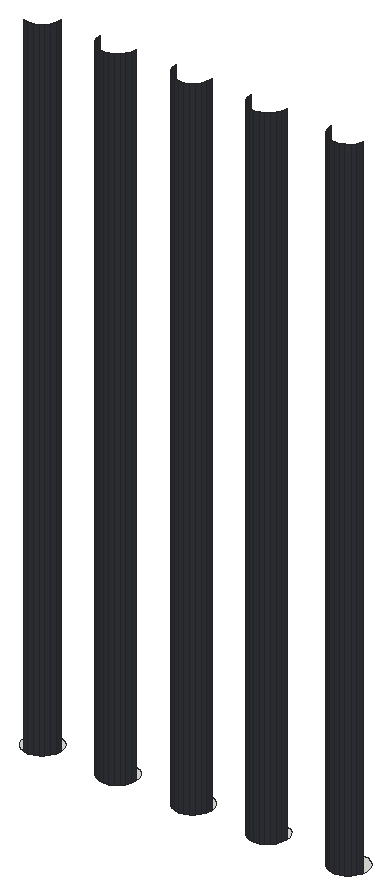
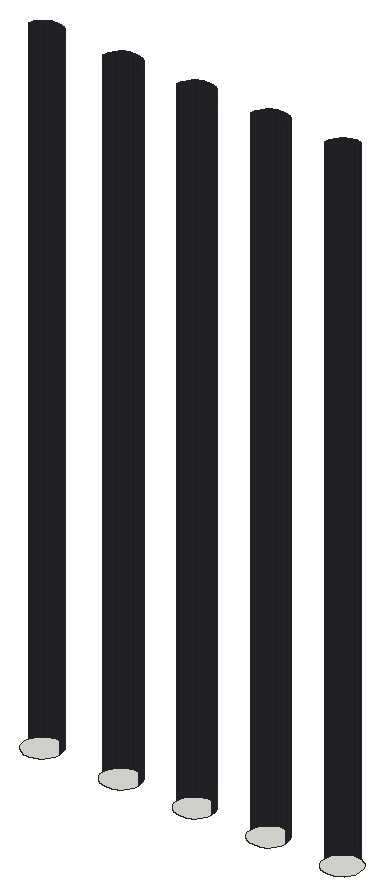
# SketchUp Ruby script. Lengths in inches.
U = 1.inch
M = Sketchup.active_model
def pt(a) = Geom::Point3d.new(a.map { |v| v * U })
def face(e, loops, mat)
  f = e.add_face(loops[0].map { |a| pt(a) })
  loops[1..].each { |l| e.add_face(l.map { |a| pt(a) }).erase! }
  f.material = f.back_material = mat if mat
  f
end
# faces: each face lists its corners as indices into pts; further lists are holes
def faces(e, pts, list, mat = nil) = list.each { |f| face(e, (f[0].is_a?(Array) ? f : [f]).map { |l| l.map { |i| pts[i] } }, mat) }
# xy, xz, yz: faces in a plane at the given z, y or x. An outline is a flat list of corners, or four numbers for a rectangle; further outlines are holes
def ring(l) = l.size == 4 ? [[l[0], l[1]], [l[2], l[1]], [l[2], l[3]], [l[0], l[3]]] : l.each_slice(2).to_a
def flat(e, list, mat, &to3) = list.each { |f| face(e, (f[0].is_a?(Array) ? f : [f]).map { |l| ring(l).map { |u, v| to3.(u, v) } }, mat) }
def xy(e, z, list, mat = nil) = flat(e, list, mat) { |x, y| [x, y, z] }
def xz(e, y, list, mat = nil) = flat(e, list, mat) { |x, z| [x, y, z] }
def yz(e, x, list, mat = nil) = flat(e, list, mat) { |y, z| [x, y, z] }
def lines(e, pts, list) = list.each { |a, b| e.add_line(pt(pts[a]), pt(pts[b])) }
# prism: a flat outline (further loops are holes) pulled along v
def prism(e, loops, v, mat = nil)
  f = face(e, loops, mat); d = Geom::Vector3d.new(v.map { |x| x * U })
  f.pushpull(f.normal.samedirection?(d) ? d.length : -d.length)
end
def box(e, o, s, mat = nil) = prism(e, [[o, [o[0] + s[0], o[1], o[2]], [o[0] + s[0], o[1] + s[1], o[2]], [o[0], o[1] + s[1], o[2]]]], [0, 0, s[2]], mat)
def at(x, y, z, deg = 0) = Geom::Transformation.translation(pt([x, y, z])) * Geom::Transformation.rotation(ORIGIN, Z_AXIS, deg.degrees)
def axes(o, x, y, z) = Geom::Transformation.new([*x, 0, *y, 0, *z, 0, *pt(o).to_a, 1])
def part(name) = M.definitions.add(name)
# library, detail: a bought-in or finely detailed component or shape, given as its bounding box
def library(name, o, s) = part(name).tap { |d| box(d.entities, o, s) }
def detail(e, o, s) = box(e.add_group.entities, o, s)
def put(e, d, t, mat = nil) = e.add_instance(d, t).tap { |i| i.material = mat if mat }
def group(e, t, mat = nil) = e.add_group.tap { |g| g.transformation = t; g.material = mat if mat }.entities
root = M.entities
M.materials.add("[Formica Laminate Dark]").color = [50, 53, 60]
xy(root,22.1875,[[172.83,106,172.65,106.02,172.49,106.09,172.35,106.2,172.24,106.34,172.17,106.51,172.15,106.6875,172.17,106.87,172.24,107.03,172.35,107.17,172.49,107.28,172.65,107.35,172.83,107.375,173.01,107.35,173.18,107.28,173.32,107.17,173.43,107.03,173.5,106.87,173.52,106.6875,173.5,106.51,173.43,106.34,173.32,106.2,173.18,106.09,173.01,106.02],[175.71,106,175.53,106.02,175.36,106.09,175.22,106.2,175.11,106.34,175.04,106.51,175.02,106.6875,175.04,106.87,175.11,107.03,175.22,107.17,175.36,107.28,175.53,107.35,175.71,107.375,175.89,107.35,176.05,107.28,176.19,107.17,176.3,107.03,176.37,106.87,176.4,106.6875,176.37,106.51,176.3,106.34,176.19,106.2,176.05,106.09,175.89,106.02],[178.58,106,178.4,106.02,178.24,106.09,178.1,106.2,177.99,106.34,177.92,106.51,177.9,106.6875,177.92,106.87,177.99,107.03,178.1,107.17,178.24,107.28,178.4,107.35,178.58,107.375,178.76,107.35,178.93,107.28,179.07,107.17,179.18,107.03,179.25,106.87,179.27,106.6875,179.25,106.51,179.18,106.34,179.07,106.2,178.93,106.09,178.76,106.02],[181.46,106,181.28,106.02,181.11,106.09,180.97,106.2,180.86,106.34,180.79,106.51,180.77,106.6875,180.79,106.87,180.86,107.03,180.97,107.17,181.11,107.28,181.28,107.35,181.46,107.375,181.64,107.35,181.8,107.28,181.94,107.17,182.05,107.03,182.12,106.87,182.15,106.6875,182.12,106.51,182.05,106.34,181.94,106.2,181.8,106.09,181.64,106.02],[184.52,106,184.34,106.02,184.18,106.09,184.03,106.2,183.92,106.34,183.86,106.51,183.83,106.6875,183.86,106.87,183.92,107.03,184.03,107.17,184.18,107.28,184.34,107.35,184.52,107.375,184.7,107.35,184.86,107.28,185.01,107.17,185.12,107.03,185.18,106.87,185.21,106.6875,185.18,106.51,185.12,106.34,185.01,106.2,184.86,106.09,184.7,106.02]])
p = [[172.65,106.02,22.1875],[172.83,106,22.1875],[172.83,106,47.21],[172.65,106.02,47.21],[173.01,106.02,22.1875],[173.01,106.02,47.21],
  [173.18,106.09,22.1875],[173.18,106.09,47.21],[175.36,106.09,22.1875],[175.53,106.02,22.1875],[175.53,106.02,47.21],[175.36,106.09,47.21],
  [175.71,106,22.1875],[175.71,106,47.21],[175.89,106.02,22.1875],[175.89,106.02,47.21],[176.05,106.09,22.1875],[176.05,106.09,47.21],
  [178.24,106.09,22.1875],[178.4,106.02,22.1875],[178.4,106.02,47.21],[178.24,106.09,47.21],[178.58,106,22.1875],[178.58,106,47.21],
  [178.76,106.02,22.1875],[178.76,106.02,47.21],[178.93,106.09,22.1875],[178.93,106.09,47.21],[181.11,106.09,22.1875],[181.28,106.02,22.1875],
  [181.28,106.02,47.21],[181.11,106.09,47.21],[181.46,106,22.1875],[181.46,106,47.21],[181.64,106.02,22.1875],[181.64,106.02,47.21],
  [181.8,106.09,22.1875],[181.8,106.09,47.21],[184.18,106.09,22.1875],[184.34,106.02,22.1875],[184.34,106.02,47.21],[184.18,106.09,47.21],
  [184.52,106,22.1875],[184.52,106,47.21],[184.7,106.02,22.1875],[184.7,106.02,47.21],[184.86,106.09,22.1875],[184.86,106.09,47.21],
  [173.32,106.2,22.1875],[173.32,106.2,47.21],[175.22,106.2,22.1875],[175.22,106.2,47.21],[176.19,106.2,22.1875],[176.19,106.2,47.21],
  [178.1,106.2,22.1875],[178.1,106.2,47.21],[179.07,106.2,22.1875],[179.07,106.2,47.21],[180.97,106.2,22.1875],[180.97,106.2,47.21],
  [181.94,106.2,22.1875],[181.94,106.2,47.21],[184.03,106.2,22.1875],[184.03,106.2,47.21],[185.01,106.2,22.1875],[185.01,106.2,47.21],
  [173.43,106.34,22.1875],[173.43,106.34,47.21],[175.11,106.34,22.1875],[175.11,106.34,47.21],[176.3,106.34,22.1875],[176.3,106.34,47.21],
  [177.99,106.34,22.1875],[177.99,106.34,47.21],[179.18,106.34,22.1875],[179.18,106.34,47.21],[180.86,106.34,22.1875],[180.86,106.34,47.21],
  [182.05,106.34,22.1875],[182.05,106.34,47.21],[183.92,106.34,22.1875],[183.92,106.34,47.21],[185.12,106.34,22.1875],[185.12,106.34,47.21],
  [173.5,106.51,22.1875],[173.5,106.51,47.21],[175.04,106.51,22.1875],[175.04,106.51,47.21],[176.37,106.51,22.1875],[176.37,106.51,47.21],
  [177.92,106.51,22.1875],[177.92,106.51,47.21],[179.25,106.51,22.1875],[179.25,106.51,47.21],[180.79,106.51,22.1875],[180.79,106.51,47.21],
  [182.12,106.51,22.1875],[182.12,106.51,47.21],[183.86,106.51,22.1875],[183.86,106.51,47.21],[185.18,106.51,22.1875],[185.18,106.51,47.21],
  [173.52,106.6875,22.1875],[173.52,106.6875,47.21],[175.02,106.6875,22.1875],[175.02,106.6875,47.21],[176.4,106.6875,22.1875],[176.4,106.6875,47.21],
  [177.9,106.6875,22.1875],[177.9,106.6875,47.21],[179.27,106.6875,22.1875],[179.27,106.6875,47.21],[180.77,106.6875,22.1875],[180.77,106.6875,47.21],
  [182.15,106.6875,22.1875],[182.15,106.6875,47.21],[183.83,106.6875,22.1875],[183.83,106.6875,47.21]]
faces(root,p,[[0,1,2,3],[1,4,5,2],[4,6,7,5],[8,9,10,11],[9,12,13,10],[12,14,15,13],[14,16,17,15],[18,19,20,21],
  [19,22,23,20],[22,24,25,23],[24,26,27,25],[28,29,30,31],[29,32,33,30],[32,34,35,33],[34,36,37,35],[38,39,40,41],
  [39,42,43,40],[42,44,45,43],[44,46,47,45],[6,48,49,7],[50,8,11,51],[16,52,53,17],[54,18,21,55],[26,56,57,27],
  [58,28,31,59],[36,60,61,37],[62,38,41,63],[46,64,65,47],[48,66,67,49],[68,50,51,69],[52,70,71,53],[72,54,55,73],
  [56,74,75,57],[76,58,59,77],[60,78,79,61],[80,62,63,81],[64,82,83,65],[66,84,85,67],[86,68,69,87],[70,88,89,71],
  [90,72,73,91],[74,92,93,75],[94,76,77,95],[78,96,97,79],[98,80,81,99],[82,100,101,83],[84,102,103,85],[104,86,87,105],
  [88,106,107,89],[108,90,91,109],[92,110,111,93],[112,94,95,113],[96,114,115,97],[116,98,99,117]],"[Formica Laminate Dark]")
